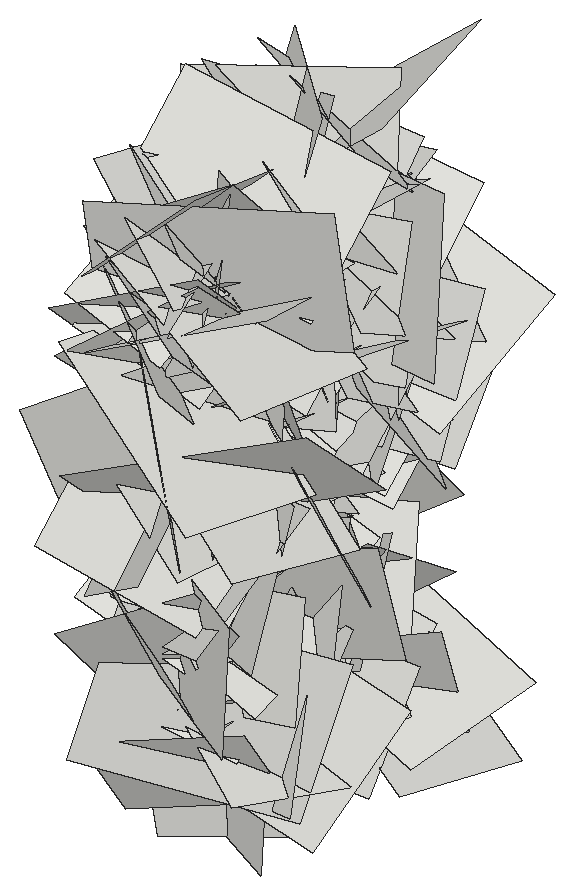
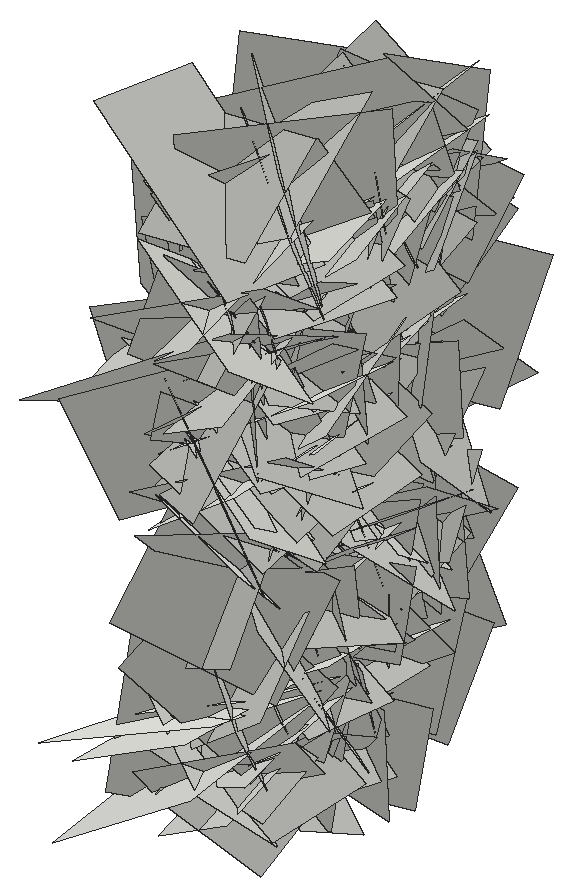
# SketchUp Ruby script. Lengths in inches.
U = 1.inch
M = Sketchup.active_model
def pt(a) = Geom::Point3d.new(a.map { |v| v * U })
def face(e, loops, mat)
  f = e.add_face(loops[0].map { |a| pt(a) })
  loops[1..].each { |l| e.add_face(l.map { |a| pt(a) }).erase! }
  f.material = f.back_material = mat if mat
  f
end
# faces: each face lists its corners as indices into pts; further lists are holes
def faces(e, pts, list, mat = nil) = list.each { |f| face(e, (f[0].is_a?(Array) ? f : [f]).map { |l| l.map { |i| pts[i] } }, mat) }
# xy, xz, yz: faces in a plane at the given z, y or x. An outline is a flat list of corners, or four numbers for a rectangle; further outlines are holes
def ring(l) = l.size == 4 ? [[l[0], l[1]], [l[2], l[1]], [l[2], l[3]], [l[0], l[3]]] : l.each_slice(2).to_a
def flat(e, list, mat, &to3) = list.each { |f| face(e, (f[0].is_a?(Array) ? f : [f]).map { |l| ring(l).map { |u, v| to3.(u, v) } }, mat) }
def xy(e, z, list, mat = nil) = flat(e, list, mat) { |x, y| [x, y, z] }
def xz(e, y, list, mat = nil) = flat(e, list, mat) { |x, z| [x, y, z] }
def yz(e, x, list, mat = nil) = flat(e, list, mat) { |y, z| [x, y, z] }
def lines(e, pts, list) = list.each { |a, b| e.add_line(pt(pts[a]), pt(pts[b])) }
# prism: a flat outline (further loops are holes) pulled along v
def prism(e, loops, v, mat = nil)
  f = face(e, loops, mat); d = Geom::Vector3d.new(v.map { |x| x * U })
  f.pushpull(f.normal.samedirection?(d) ? d.length : -d.length)
end
def box(e, o, s, mat = nil) = prism(e, [[o, [o[0] + s[0], o[1], o[2]], [o[0] + s[0], o[1] + s[1], o[2]], [o[0], o[1] + s[1], o[2]]]], [0, 0, s[2]], mat)
def at(x, y, z, deg = 0) = Geom::Transformation.translation(pt([x, y, z])) * Geom::Transformation.rotation(ORIGIN, Z_AXIS, deg.degrees)
def axes(o, x, y, z) = Geom::Transformation.new([*x, 0, *y, 0, *z, 0, *pt(o).to_a, 1])
def part(name) = M.definitions.add(name)
# library, detail: a bought-in or finely detailed component or shape, given as its bounding box
def library(name, o, s) = part(name).tap { |d| box(d.entities, o, s) }
def detail(e, o, s) = box(e.add_group.entities, o, s)
def put(e, d, t, mat = nil) = e.add_instance(d, t).tap { |i| i.material = mat if mat }
def group(e, t, mat = nil) = e.add_group.tap { |g| g.transformation = t; g.material = mat if mat }.entities
root = M.entities
c1 = part("Component\#6")
p = [[0.01,0,0],[0,3.24,4.54],[4.32,3.24,4.54],[4.33,0,0]]
faces(c1.entities,p,[[0,1,2,3]])
put(root,c1,axes([38.11,196.19,13.89],[0.03711,0.95345,-0.08325],[-0.1071,-0.07916,-0.94908],[-1.00884,0.04348,0.09769]))
put(root,c1,axes([38.11,197.24,20.32],[-0.11105,0.4932,0.81979],[0.10012,0.82599,-0.48487],[-1.00916,0.02768,-0.13831]))
put(root,c1,axes([34.14,202.56,19.21],[0.06396,-0.26998,-0.58675],[-0.04641,-0.58965,0.26682],[0.68306,-0.01478,0.07307]))
put(root,c1,axes([34.14,199.64,2.06],[-0.21894,0.61345,0.59822],[0.01858,0.61825,-0.62794],[0.90807,0.13525,0.15708]))
put(root,c1,axes([38.11,196.07,8.125],[-0.08332,-0.69698,-0.457],[-0.10667,-0.44773,0.70016],[-0.87699,0.12068,-0.04174]))
put(root,c1,axes([34.14,190.79,19.57],[0.04866,0.55121,0.30162],[0.00575,0.30207,-0.55285],[0.66601,-0.04288,-0.01726]))
put(root,c1,axes([34.14,195.85,11.01],[-0.15114,0.73817,0.19544],[0.07767,0.21113,-0.74396],[0.80568,0.11812,0.10838]))
put(root,c1,axes([38.11,202.76,13.17],[0.11284,-1.03894,-0.17524],[-0.03066,-0.17895,1.04335],[-1.11641,-0.1001,-0.04636]))
put(root,c1,axes([38.11,189.31,11.46],[-0.01967,0.80876,0.77653],[0.21901,0.76581,-0.79265],[-1.16812,0.12996,-0.16169]))
put(root,c1,axes([34.14,193.57,4.75],[0.0218,0.6351,0.02763],[0.03876,0.02642,-0.63443],[0.67273,-0.0221,0.03566]))
put(root,c1,axes([38.11,199.68,18.17],[0.10811,0.81171,0.57509],[-0.11351,0.5837,-0.80488],[-1.04835,0.0205,0.14645]))
put(root,c1,axes([34.14,202.9,8.46],[-0.28421,-0.45126,-0.90988],[-0.10984,-0.92399,0.48879],[1.07096,-0.21452,-0.19133]))
put(root,c1,axes([34.14,193.91,15.9375],[0.03263,0.61645,-0.26034],[-0.02336,-0.25954,-0.61716],[0.70894,-0.03692,-0.00835]))
put(root,c1,axes([34.14,192.26,20.51],[-0.14395,0.6641,-0.62024],[-0.10915,-0.63433,-0.65665],[0.95701,0.02754,-0.16819]))
put(root,c1,axes([34.14,199.23,1.1],[-0.00098,-0.71414,-0.15761],[-0.04174,-0.15733,0.71311],[0.77408,-0.00939,0.03826]))
put(root,c1,axes([34.14,196.5625,6.92],[0.07674,-0.09799,-0.6482],[-0.03176,-0.65195,0.09521],[0.69417,-0.019,0.07601]))
put(root,c1,axes([34.14,198.91,12.75],[-0.15355,-0.10183,1.00426],[-0.21738,0.99636,0.07145],[1.04766,0.19182,0.16201]))
put(root,c1,axes([34.14,195.68,15.75],[0.06715,-0.51242,0.33521],[0.05381,0.34023,0.51051],[0.64683,0.02489,-0.07727]))
put(root,c1,axes([34.14,200.4375,8.06],[-0.17377,0.75884,-0.49804],[-0.05898,-0.51355,-0.76415],[0.96033,0.10576,-0.13705]))
put(root,c1,axes([34.14,199.6875,17.84],[0.07891,0.44569,0.39814],[0.07493,0.39183,-0.45185],[0.62903,-0.10259,0.00388]))
put(root,c1,axes([34.14,200.03,9.27],[-0.00412,-0.60297,0.30435],[0.07057,0.30253,0.60022],[0.71247,-0.03345,-0.05769]))
put(root,c1,axes([34.14,192.95,10.8],[0.02962,0.02518,0.78508],[-0.12702,0.77652,-0.02064],[0.82287,0.11896,-0.03145]))
put(root,c1,axes([38.11,199.37,10.67],[0.09558,-1.01864,0.46326],[0.13943,0.47118,1.01047],[-1.17795,-0.02688,0.1572]))
put(root,c1,axes([34.14,198.38,4.95],[-0.02223,0.32868,-0.55446],[0.17267,-0.53404,-0.32274],[0.66105,0.15055,0.06565]))
put(root,c1,axes([34.14,192.04,10.01],[-0.12172,0.5206,-0.6372],[0.01939,-0.6416,-0.52749],[0.87198,0.08694,-0.07722]))
put(root,c1,axes([34.14,202.51,19.98],[0.06792,0.48446,-0.5602],[-0.10116,-0.55221,-0.48846],[0.77852,-0.11402,-0.01459]))
put(root,c1,axes([38.11,195.86,16.68],[-0.06531,-0.43873,0.684],[-0.07025,0.68639,0.43429],[-0.8585,-0.02279,-0.08757]))
put(root,c1,axes([34.14,202.74,-0.14],[0.03158,-0.64507,0.25861],[0.01592,0.25938,0.64528],[0.73651,0.02205,-0.02503]))
put(root,c1,axes([38.11,192.22,20.81],[-0.00161,0.62306,-0.59539],[-0.0785,-0.59329,-0.62067],[-0.91013,0.05007,0.05459]))
put(root,c1,axes([34.14,197.35,3.52],[0.03443,0.41092,0.66217],[-0.08038,0.66126,-0.40665],[0.82215,0.04744,-0.06748]))
put(root,c1,axes([34.14,195.99,4.23],[-0.18601,0.0566,0.88651],[0.05201,0.90288,-0.04793],[0.94017,-0.03875,0.17804]))
put(root,c1,axes([38.11,198.67,11.97],[0.07539,0.76068,0.50866],[-0.0723,0.51318,-0.75791],[-0.96729,0.02092,0.0963]))
put(root,c1,axes([34.14,195.9375,9.16],[0.07841,0.69576,-0.29748],[-0.09095,-0.28926,-0.69787],[0.79692,-0.10147,-0.05038]))
put(root,c1,axes([38.11,195.4375,18.11],[-0.16874,-0.51977,-0.57708],[0.05885,-0.59519,0.52076],[-0.82114,0.06415,0.15591]))
put(root,c1,axes([38.11,196.17,12.88],[0.06274,0.02618,0.84664],[-0.15393,0.83645,-0.01571],[-0.88457,-0.1437,0.06278]))
put(root,c1,axes([38.11,193.46,10.77],[-0.10152,0.90556,-0.18731],[0.17799,-0.16815,-0.89879],[-0.96391,-0.12642,-0.14624]))
put(root,c1,axes([34.14,200.82,0.59],[0.02153,-0.73416,-0.35765],[-0.0933,-0.35764,0.72915],[0.8606,-0.02041,0.08799]))
put(root,c1,axes([38.11,195.73,16.63],[0.01219,-0.78698,0.32297],[-0.05977,0.32158,0.78561],[-0.89973,-0.03203,-0.04781]))
put(root,c1,axes([38.11,196.375,20.79],[0.12547,0.87042,-0.10702],[-0.18806,-0.08199,-0.86307],[-0.91037,0.1369,0.16354]))
put(root,c1,axes([38.11,200.05,13.66],[-0.07814,0.81604,-0.08962],[0.02759,-0.08761,-0.81916],[-0.86976,-0.0761,-0.01794]))
put(root,c1,axes([38.11,198.3125,4.47],[0.08144,0.93817,-0.09306],[0.01009,-0.09413,-0.94116],[-0.99929,0.07551,-0.01709]))
put(root,c1,axes([38.11,200.41,3.58],[0.05776,-0.87144,-0.04483],[-0.06577,-0.04867,0.87073],[-0.92261,-0.05109,-0.06488]))
put(root,c1,axes([38.11,195.95,14.86],[0.17446,0.9838,0.62037],[0.19333,0.59697,-0.99508],[-1.2176,0.23574,-0.06911]))
put(root,c1,axes([38.11,194.43,21.03],[0.18864,1.08922,-0.2367],[0.12278,-0.25647,-1.09312],[-1.17512,0.14806,-0.15221]))
put(root,c1,axes([34.14,200.69,6.875],[-0.16125,-0.91938,-0.30199],[-0.04119,-0.29965,0.93182],[1.02494,-0.15668,-0.01006]))
put(root,c1,axes([38.11,193.09,19.46],[-0.07295,0.25641,0.83596],[0.12348,0.83376,-0.24615],[-0.9186,0.09171,-0.09948]))
put(root,c1,axes([38.11,196.25,20.97],[-0.03433,0.46285,-0.75346],[0.09275,-0.74858,-0.46362],[-0.93272,-0.09148,-0.01837]))
put(root,c1,axes([34.14,193.9,23.36],[0.05376,0.55183,-0.55937],[-0.04326,-0.55793,-0.55411],[0.83178,-0.06469,0.00734]))
put(root,c1,axes([38.11,193.92,18.08],[0.13809,0.41624,-1.10581],[0.27382,-1.09563,-0.38198],[-1.22215,-0.19844,-0.21052]))
put(root,c1,axes([38.11,202.38,16.09],[0.07402,-0.92988,-0.45649],[0.17154,-0.44211,0.92536],[-1.08456,-0.13339,0.1152]))
put(root,c1,axes([34.14,201.99,11.3125],[-0.07595,0.62186,-0.76254],[-0.14567,-0.76339,-0.60964],[1.03278,-0.06194,-0.14206]))
put(root,c1,axes([34.14,202.11,15.27],[0.00741,-0.76642,-0.19435],[0.02033,-0.19414,0.76626],[0.83787,0.01149,-0.01688]))
put(root,c1,axes([38.11,195.27,-1.16],[0.10176,-0.07093,0.82892],[-0.16666,0.81783,0.08819],[-0.86597,-0.16573,0.08043]))
put(root,c1,axes([38.11,196.11,19.5625],[0.1708,0.27531,1.11719],[0.21419,1.10379,-0.30115],[-1.2007,0.23607,0.1052]))
put(root,c1,axes([34.14,200.46,4.14],[0.03987,0.66432,-0.22968],[0.12809,-0.2327,-0.65325],[0.73398,0.00452,0.12648]))
put(root,c1,axes([38.11,200.85,9.74],[-0.02518,0.49854,0.49521],[-0.19267,0.47427,-0.48618],[-0.7195,-0.14445,0.11286]))
put(root,c1,axes([34.14,192.1875,23.6],[0.04344,0.89705,-0.17333],[-0.1764,-0.16328,-0.88435],[0.95226,-0.07116,-0.15591]))
put(root,c1,axes([38.11,192.1875,23.6],[-0.04344,0.89705,-0.17333],[0.1764,-0.16328,-0.88435],[-0.95226,-0.07116,-0.15591]))
put(root,c1,axes([34.14,200.85,9.74],[0.02518,0.49854,0.49521],[0.19267,0.47427,-0.48618],[0.7195,-0.14445,0.11286]))
put(root,c1,axes([38.11,200.46,4.14],[-0.03987,0.66432,-0.22968],[-0.12809,-0.2327,-0.65325],[-0.73398,0.00452,0.12648]))
put(root,c1,axes([34.14,196.11,19.5625],[-0.1708,0.27531,1.11719],[-0.21419,1.10379,-0.30115],[1.2007,0.23607,0.1052]))
put(root,c1,axes([34.14,195.27,-1.16],[-0.10176,-0.07093,0.82892],[0.16666,0.81783,0.08819],[0.86597,-0.16573,0.08043]))
put(root,c1,axes([38.11,202.11,15.27],[-0.00741,-0.76642,-0.19435],[-0.02033,-0.19414,0.76626],[-0.83787,0.01149,-0.01688]))
put(root,c1,axes([38.11,201.99,11.3125],[0.07595,0.62186,-0.76254],[0.14567,-0.76339,-0.60964],[-1.03278,-0.06194,-0.14206]))
put(root,c1,axes([34.14,202.38,16.09],[-0.07402,-0.92988,-0.45649],[-0.17154,-0.44211,0.92536],[1.08456,-0.13339,0.1152]))
put(root,c1,axes([34.14,193.92,18.08],[-0.13809,0.41624,-1.10581],[-0.27382,-1.09563,-0.38198],[1.22215,-0.19844,-0.21052]))
put(root,c1,axes([38.11,193.9,23.36],[-0.05376,0.55183,-0.55937],[0.04326,-0.55793,-0.55411],[-0.83178,-0.06469,0.00734]))
put(root,c1,axes([34.14,196.25,20.97],[0.03433,0.46285,-0.75346],[-0.09275,-0.74858,-0.46362],[0.93272,-0.09148,-0.01837]))
put(root,c1,axes([34.14,193.09,19.46],[0.07295,0.25641,0.83596],[-0.12348,0.83376,-0.24615],[0.9186,0.09171,-0.09948]))
put(root,c1,axes([38.11,200.69,6.875],[0.16125,-0.91938,-0.30199],[0.04119,-0.29965,0.93182],[-1.02494,-0.15668,-0.01006]))
put(root,c1,axes([34.14,194.43,21.03],[-0.18864,1.08922,-0.2367],[-0.12278,-0.25647,-1.09312],[1.17512,0.14806,-0.15221]))
put(root,c1,axes([34.14,195.95,14.86],[-0.17446,0.9838,0.62037],[-0.19333,0.59697,-0.99508],[1.2176,0.23574,-0.06911]))
put(root,c1,axes([34.14,200.41,3.58],[-0.05776,-0.87144,-0.04483],[0.06577,-0.04867,0.87073],[0.92261,-0.05109,-0.06488]))
put(root,c1,axes([34.14,198.3125,4.47],[-0.08144,0.93817,-0.09306],[-0.01009,-0.09413,-0.94116],[0.99929,0.07551,-0.01709]))
put(root,c1,axes([34.14,200.05,13.66],[0.07814,0.81604,-0.08962],[-0.02759,-0.08761,-0.81916],[0.86976,-0.0761,-0.01794]))
put(root,c1,axes([34.14,196.375,20.79],[-0.12547,0.87042,-0.10702],[0.18806,-0.08199,-0.86307],[0.91037,0.1369,0.16354]))
put(root,c1,axes([34.14,195.73,16.63],[-0.01219,-0.78698,0.32297],[0.05977,0.32158,0.78561],[0.89973,-0.03203,-0.04781]))
put(root,c1,axes([38.11,200.82,0.59],[-0.02153,-0.73416,-0.35765],[0.0933,-0.35764,0.72915],[-0.8606,-0.02041,0.08799]))
put(root,c1,axes([34.14,193.46,10.77],[0.10152,0.90556,-0.18731],[-0.17799,-0.16815,-0.89879],[0.96391,-0.12642,-0.14624]))
put(root,c1,axes([34.14,196.17,12.88],[-0.06274,0.02618,0.84664],[0.15393,0.83645,-0.01571],[0.88457,-0.1437,0.06278]))
put(root,c1,axes([34.14,195.4375,18.11],[0.16874,-0.51977,-0.57708],[-0.05885,-0.59519,0.52076],[0.82114,0.06415,0.15591]))
put(root,c1,axes([38.11,195.9375,9.16],[-0.07841,0.69576,-0.29748],[0.09095,-0.28926,-0.69787],[-0.79692,-0.10147,-0.05038]))
put(root,c1,axes([34.14,198.67,11.97],[-0.07539,0.76068,0.50866],[0.0723,0.51318,-0.75791],[0.96729,0.02092,0.0963]))
put(root,c1,axes([38.11,195.99,4.23],[0.18601,0.0566,0.88651],[-0.05201,0.90288,-0.04793],[-0.94017,-0.03875,0.17804]))
put(root,c1,axes([38.11,197.35,3.52],[-0.03443,0.41092,0.66217],[0.08038,0.66126,-0.40665],[-0.82215,0.04744,-0.06748]))
put(root,c1,axes([34.14,192.22,20.81],[0.00161,0.62306,-0.59539],[0.0785,-0.59329,-0.62067],[0.91013,0.05007,0.05459]))
put(root,c1,axes([38.11,202.74,-0.14],[-0.03158,-0.64507,0.25861],[-0.01592,0.25938,0.64528],[-0.73651,0.02205,-0.02503]))
put(root,c1,axes([34.14,195.86,16.68],[0.06531,-0.43873,0.684],[0.07025,0.68639,0.43429],[0.8585,-0.02279,-0.08757]))
put(root,c1,axes([38.11,202.51,19.98],[-0.06792,0.48446,-0.5602],[0.10116,-0.55221,-0.48846],[-0.77852,-0.11402,-0.01459]))
put(root,c1,axes([38.11,192.04,10.01],[0.12172,0.5206,-0.6372],[-0.01939,-0.6416,-0.52749],[-0.87198,0.08694,-0.07722]))
put(root,c1,axes([38.11,198.38,4.95],[0.02223,0.32868,-0.55446],[-0.17267,-0.53404,-0.32274],[-0.66105,0.15055,0.06565]))
put(root,c1,axes([34.14,199.37,10.67],[-0.09558,-1.01864,0.46326],[-0.13943,0.47118,1.01047],[1.17795,-0.02688,0.1572]))
put(root,c1,axes([38.11,192.95,10.8],[-0.02962,0.02518,0.78508],[0.12702,0.77652,-0.02064],[-0.82287,0.11896,-0.03145]))
put(root,c1,axes([38.11,200.03,9.27],[0.00412,-0.60297,0.30435],[-0.07057,0.30253,0.60022],[-0.71247,-0.03345,-0.05769]))
put(root,c1,axes([38.11,199.6875,17.84],[-0.07891,0.44569,0.39814],[-0.07493,0.39183,-0.45185],[-0.62903,-0.10259,0.00388]))
put(root,c1,axes([38.11,200.4375,8.06],[0.17377,0.75884,-0.49804],[0.05898,-0.51355,-0.76415],[-0.96033,0.10576,-0.13705]))
put(root,c1,axes([38.11,195.68,15.75],[-0.06715,-0.51242,0.33521],[-0.05381,0.34023,0.51051],[-0.64683,0.02489,-0.07727]))
put(root,c1,axes([38.11,198.91,12.75],[0.15355,-0.10183,1.00426],[0.21738,0.99636,0.07145],[-1.04766,0.19182,0.16201]))
put(root,c1,axes([38.11,196.5625,6.92],[-0.07674,-0.09799,-0.6482],[0.03176,-0.65195,0.09521],[-0.69417,-0.019,0.07601]))
put(root,c1,axes([38.11,199.23,1.1],[0.00098,-0.71414,-0.15761],[0.04174,-0.15733,0.71311],[-0.77408,-0.00939,0.03826]))
put(root,c1,axes([38.11,192.26,20.51],[0.14395,0.6641,-0.62024],[0.10915,-0.63433,-0.65665],[-0.95701,0.02754,-0.16819]))
put(root,c1,axes([38.11,193.91,15.9375],[-0.03263,0.61645,-0.26034],[0.02336,-0.25954,-0.61716],[-0.70894,-0.03692,-0.00835]))
put(root,c1,axes([38.11,202.9,8.46],[0.28421,-0.45126,-0.90988],[0.10984,-0.92399,0.48879],[-1.07096,-0.21452,-0.19133]))
put(root,c1,axes([34.14,199.68,18.17],[-0.10811,0.81171,0.57509],[0.11351,0.5837,-0.80488],[1.04835,0.0205,0.14645]))
put(root,c1,axes([38.11,193.57,4.75],[-0.0218,0.6351,0.02763],[-0.03876,0.02642,-0.63443],[-0.67273,-0.0221,0.03566]))
put(root,c1,axes([34.14,189.31,11.46],[0.01967,0.80876,0.77653],[-0.21901,0.76581,-0.79265],[1.16812,0.12996,-0.16169]))
put(root,c1,axes([34.14,202.76,13.17],[-0.11284,-1.03894,-0.17524],[0.03066,-0.17895,1.04335],[1.11641,-0.1001,-0.04636]))
put(root,c1,axes([38.11,195.85,11.01],[0.15114,0.73817,0.19544],[-0.07767,0.21113,-0.74396],[-0.80568,0.11812,0.10838]))
put(root,c1,axes([38.11,190.79,19.57],[-0.04866,0.55121,0.30162],[-0.00575,0.30207,-0.55285],[-0.66601,-0.04288,-0.01726]))
put(root,c1,axes([34.14,196.07,8.125],[0.08332,-0.69698,-0.457],[0.10667,-0.44773,0.70016],[0.87699,0.12068,-0.04174]))
put(root,c1,axes([38.11,199.64,2.06],[0.21894,0.61345,0.59822],[-0.01858,0.61825,-0.62794],[-0.90807,0.13525,0.15708]))
put(root,c1,axes([38.11,202.56,19.21],[-0.06396,-0.26998,-0.58675],[0.04641,-0.58965,0.26682],[-0.68306,-0.01478,0.07307]))
put(root,c1,axes([34.14,197.24,20.32],[0.11105,0.4932,0.81979],[-0.10012,0.82599,-0.48487],[1.00916,0.02768,-0.13831]))
put(root,c1,axes([34.14,196.19,13.89],[-0.03711,0.95345,-0.08325],[0.1071,-0.07916,-0.94908],[1.00884,0.04348,0.09769]))
put(root,c1,axes([38.11,198.53,13.8],[0.10676,-0.41647,0.70694],[0.09382,0.7136,0.40779],[-0.86465,0.02601,0.13154]))
put(root,c1,axes([38.11,201.03,8.02],[0.03451,-0.61291,-0.20918],[-0.0475,-0.21108,0.61149],[-0.68484,-0.01625,-0.05296]))
put(root,c1,axes([38.11,199.53,17.66],[0.07108,0.22718,0.77768],[0.14032,0.76678,-0.23541],[-0.84726,0.14605,0.02626]))
put(root,c1,axes([38.11,196.1,5.28],[0.08762,-0.56519,-0.39893],[-0.0287,-0.4041,0.56691],[-0.73275,-0.05175,-0.06991]))
put(root,c1,axes([34.14,192.44,8.79],[-0.05887,1.04295,0.25043],[0.00297,0.2509,-1.04431],[1.13694,0.05335,0.0157]))
put(root,c1,axes([34.14,193.71,0.46],[0.00413,-0.52236,0.7551],[0.18121,0.74232,0.51263],[0.95624,-0.13842,-0.10041]))
put(root,c1,axes([34.14,195.28,4.79],[0.03702,0.87634,0.85063],[-0.28559,0.83554,-0.84973],[1.26267,0.16329,-0.21713]))
put(root,c1,axes([34.14,203.91,5.3125],[0.18463,-0.58129,-0.78091],[-0.13848,-0.80009,0.56643],[1.02258,-0.00339,0.2177]))
put(root,c1,axes([34.14,198.93,5.125],[0.08676,0.85287,0.14934],[0.16568,0.13299,-0.84515],[0.90272,-0.10637,0.14076]))
put(root,c1,axes([34.14,198.84,9.75],[-0.24721,-0.9594,-0.88495],[-0.06038,-0.89063,0.98057],[1.38221,-0.2105,-0.11544]))
put(root,c1,axes([34.14,202.1,18.26],[-0.1919,-1.13475,-0.09678],[0.16378,-0.12156,1.13628],[1.19604,-0.16542,-0.17113]))
put(root,c1,axes([38.11,194.11,10.49],[0.01019,-0.66626,0.06574],[0.1187,0.06642,0.65679],[-0.69967,0.00157,0.11238]))
put(root,c1,axes([34.14,200.51,5.45],[-0.07717,-0.59417,-0.91785],[0.09928,-0.91989,0.58806],[1.15472,0.03938,-0.1119]))
put(root,c1,axes([34.14,205.24,14.9],[-0.1168,-0.46047,-1.13614],[-0.0362,-1.13913,0.465],[1.29896,-0.07315,-0.0892]))
put(root,c1,axes([34.14,194.25,1.05],[0.1707,-0.55728,0.79671],[-0.04122,0.80323,0.5697],[1.02978,0.12452,-0.10926]))
put(root,c1,axes([34.14,194.35,10.5],[-0.1187,0.07765,-1.12146],[0.14385,-1.11784,-0.09095],[1.18288,0.14373,-0.10148]))
put(root,c1,axes([34.14,197.36,24.8],[-0.09794,1.0389,-0.68546],[-0.01654,-0.68826,-1.04104],[1.31923,0.0685,-0.06394]))
put(root,c1,axes([38.11,199.74,12.37],[0.13977,-0.41949,-0.41774],[-0.0557,-0.43458,0.41982],[-0.62506,-0.05508,-0.13082]))
put(root,c1,axes([38.11,199.42,15.6],[0.03605,-0.49998,-0.38134],[0.14474,-0.36691,0.49324],[-0.65063,-0.10932,0.0886]))
put(root,c1,axes([34.14,200.08,24.34],[0.03463,0.75517,-0.67877],[0.20748,-0.67107,-0.73718],[1.05612,0.10708,0.16708]))
put(root,c1,axes([34.14,199.09,16.39],[0.13116,-1.14374,0.05938],[-0.13174,0.04596,1.1443],[1.20683,0.12933,0.11846]))
put(root,c1,axes([34.14,192.66,5.0625],[0.03803,0.06475,1.02957],[0.25075,1.00223,-0.07127],[1.06436,-0.23842,-0.02]))
put(root,c1,axes([34.14,196.53,2.03],[0.14871,0.38131,0.94323],[0.09041,0.94439,-0.39446],[1.07463,-0.13222,-0.09734]))
put(root,c1,axes([34.14,200.2,14.91],[0.20407,-0.96139,-0.18597],[0.07393,-0.17559,0.97991],[1.03533,0.20204,-0.03331]))
put(root,c1,axes([34.14,198.375,11.05],[-0.00636,-0.47599,-1.14741],[-0.03555,-1.14695,0.47597],[1.31628,-0.03327,0.00731]))
put(root,c1,axes([34.14,202.25,12.93],[-0.19135,-1.27912,0.12446],[0.2118,0.09622,1.27869],[1.34571,-0.19703,-0.18355]))
put(root,c1,axes([34.14,197.86,18.23],[0.19608,0.2602,-1.0463],[-0.01915,-1.06069,-0.26697],[1.14269,-0.06243,0.17507]))
put(root,c1,axes([34.14,197.84,4.84],[0.11369,-0.36766,-0.96616],[0.19069,-0.94989,0.38144],[1.07906,0.2066,0.03439]))
put(root,c1,axes([34.14,200.375,7.61],[0.26418,-0.51362,-0.84712],[0.05211,-0.86603,0.53955],[1.04881,0.1724,0.18657]))
put(root,c1,axes([34.14,203.04,12.11],[0.14841,-0.94408,-0.5752],[0.05434,-0.57362,0.95398],[1.17058,0.14632,0.02864]))
put(root,c1,axes([34.14,199.56,18.73],[0.07364,1.07871,-0.62029],[-0.05176,-0.61841,-1.08091],[1.31797,-0.08456,-0.00779]))
put(root,c1,axes([34.14,204.42,20.53],[0.1154,-1.25003,-0.28156],[-0.14973,-0.29256,1.24425],[1.34995,0.07441,0.16208]))
put(root,c1,axes([34.14,195.93,15.54],[0.04965,0.25406,1.2028],[0.02984,1.20314,-0.25523],[1.30276,-0.03724,-0.03999]))
put(root,c1,axes([34.14,198.85,12.57],[0.15345,0.48368,1.12599],[-0.09378,1.13498,-0.47617],[1.29562,0.02486,-0.16783]))
put(root,c1,axes([34.14,200.7,5.85],[0.20906,1.0682,-0.14016],[0.07965,-0.15578,-1.08152],[1.13921,-0.18514,0.10133]))
put(root,c1,axes([34.14,194.09,6.34],[0.25898,1.07168,-0.21064],[-0.01285,-0.21318,-1.09862],[1.15764,-0.24212,0.03493]))
put(root,c1,axes([34.14,192.7,21.39],[0.08893,0.79245,0.9015],[0.06254,0.89988,-0.79652],[1.27076,-0.09974,-0.02389]))
put(root,c1,axes([34.14,199.38,-0.0625],[0.15183,-0.50198,1.07326],[0.00307,1.08122,0.50532],[1.25594,0.05804,-0.13098]))
put(root,c1,axes([34.14,200.25,4.79],[0.06637,1.27776,-0.24675],[-0.01199,-0.2465,-1.2793],[1.3794,-0.06362,0.00075]))
put(root,c1,axes([34.14,192.73,15.73],[0.12897,1.2724,-0.23633],[-0.08155,-0.22984,-1.27707],[1.36939,-0.13352,-0.05379]))
put(root,c1,axes([34.14,200.21,21.54],[0.14018,1.21556,-0.55877],[-0.14242,-0.54659,-1.22085],[1.41094,-0.17594,-0.06772]))
put(root,c1,axes([34.14,190.45,18.05],[0.16537,1.24759,-0.14593],[-0.05265,-0.14081,-1.25691],[1.33042,-0.16065,-0.0316]))
put(root,c1,axes([34.14,190.86,3.39],[0.21383,0.32739,1.20741],[-0.09698,1.22359,-0.31649],[1.32251,0.03679,-0.21843]))
put(root,c1,axes([34.14,195.52,16.87],[0.17814,-1.09516,0.21581],[0.19304,0.24222,1.08736],[1.16734,0.12707,-0.21275]))
put(root,c1,axes([34.14,201.79,17.38],[0.19939,0.73728,-1.06028],[-0.09629,-1.06126,-0.75408],[1.36551,-0.18249,0.10164]))
put(root,c1,axes([34.14,196.26,4.8],[0.10051,-0.43998,1.12809],[0.21352,1.12151,0.42048],[1.26562,-0.15427,-0.16053]))
put(root,c1,axes([34.14,191.67,21.5],[0.0579,1.33618,-0.15223],[0.05318,-0.15428,-1.33612],[1.42453,-0.04855,0.05606]))
put(root,c1,axes([34.14,198.6875,16.83],[0.02201,1.26014,0.56955],[0.0456,0.56875,-1.25994],[1.46513,-0.03663,0.03065]))
put(root,c1,axes([34.14,196.95,13.22],[0.12152,0.35472,1.26895],[0.01769,1.27325,-0.35743],[1.39654,-0.047,-0.10589]))
put(root,c1,axes([34.14,197.84,15.77],[0.08558,0.66637,-1.22765],[0.01617,-1.23004,-0.66667],[1.48057,-0.02508,0.07824]))
put(root,c1,axes([34.14,193.34,3.5],[0.3285,0.68164,0.95344],[0.04901,0.97833,-0.71446],[1.2414,-0.219,-0.22409]))
put(root,c1,axes([34.14,192.59,17.15],[0.08597,-0.32374,1.28455],[0.18245,1.27862,0.31138],[1.3923,-0.14756,-0.12012]))
put(root,c1,axes([34.14,199.09,4.9],[0.11121,1.25407,0.182],[0.25083,0.16003,-1.23904],[1.31962,-0.1361,0.22018]))
put(root,c1,axes([34.14,194.4,9.86],[0.11876,-1.04596,0.91618],[0.1474,0.92297,1.03671],[1.46651,-0.00807,-0.1784]))
put(root,c1,axes([34.14,202.95,19.72],[0.19445,-0.3512,-1.29554],[0.25274,-1.27827,0.38028],[1.40021,0.2795,0.11127]))
